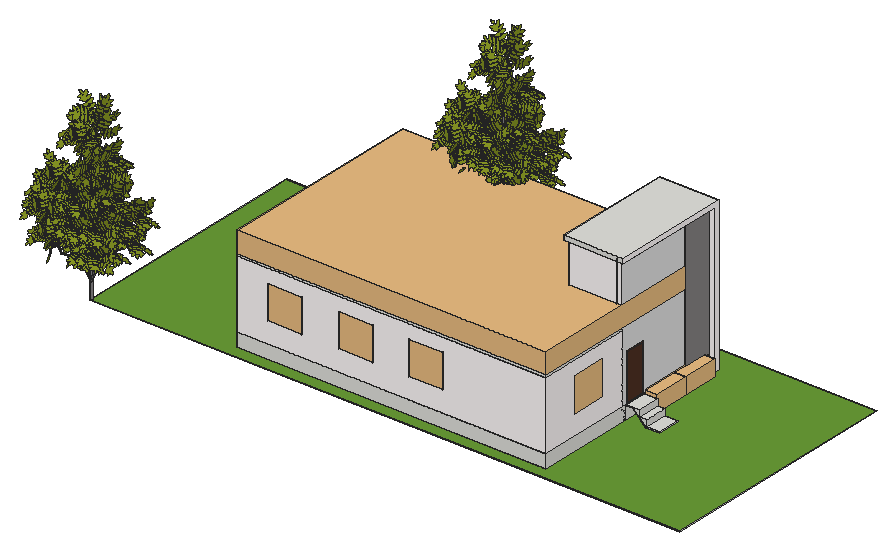
# SketchUp Ruby script. Lengths in inches.
U = 1.inch
M = Sketchup.active_model
def pt(a) = Geom::Point3d.new(a.map { |v| v * U })
def face(e, loops, mat)
  f = e.add_face(loops[0].map { |a| pt(a) })
  loops[1..].each { |l| e.add_face(l.map { |a| pt(a) }).erase! }
  f.material = f.back_material = mat if mat
  f
end
# faces: each face lists its corners as indices into pts; further lists are holes
def faces(e, pts, list, mat = nil) = list.each { |f| face(e, (f[0].is_a?(Array) ? f : [f]).map { |l| l.map { |i| pts[i] } }, mat) }
# xy, xz, yz: faces in a plane at the given z, y or x. An outline is a flat list of corners, or four numbers for a rectangle; further outlines are holes
def ring(l) = l.size == 4 ? [[l[0], l[1]], [l[2], l[1]], [l[2], l[3]], [l[0], l[3]]] : l.each_slice(2).to_a
def flat(e, list, mat, &to3) = list.each { |f| face(e, (f[0].is_a?(Array) ? f : [f]).map { |l| ring(l).map { |u, v| to3.(u, v) } }, mat) }
def xy(e, z, list, mat = nil) = flat(e, list, mat) { |x, y| [x, y, z] }
def xz(e, y, list, mat = nil) = flat(e, list, mat) { |x, z| [x, y, z] }
def yz(e, x, list, mat = nil) = flat(e, list, mat) { |y, z| [x, y, z] }
def lines(e, pts, list) = list.each { |a, b| e.add_line(pt(pts[a]), pt(pts[b])) }
# prism: a flat outline (further loops are holes) pulled along v
def prism(e, loops, v, mat = nil)
  f = face(e, loops, mat); d = Geom::Vector3d.new(v.map { |x| x * U })
  f.pushpull(f.normal.samedirection?(d) ? d.length : -d.length)
end
def box(e, o, s, mat = nil) = prism(e, [[o, [o[0] + s[0], o[1], o[2]], [o[0] + s[0], o[1] + s[1], o[2]], [o[0], o[1] + s[1], o[2]]]], [0, 0, s[2]], mat)
def at(x, y, z, deg = 0) = Geom::Transformation.translation(pt([x, y, z])) * Geom::Transformation.rotation(ORIGIN, Z_AXIS, deg.degrees)
def axes(o, x, y, z) = Geom::Transformation.new([*x, 0, *y, 0, *z, 0, *pt(o).to_a, 1])
def part(name) = M.definitions.add(name)
# library, detail: a bought-in or finely detailed component or shape, given as its bounding box
def library(name, o, s) = part(name).tap { |d| box(d.entities, o, s) }
def detail(e, o, s) = box(e.add_group.entities, o, s)
def put(e, d, t, mat = nil) = e.add_instance(d, t).tap { |i| i.material = mat if mat }
def group(e, t, mat = nil) = e.add_group.tap { |g| g.transformation = t; g.material = mat if mat }.entities
root = M.entities
M.materials.add("3D66_SU_1574822641685_001").color = [135, 150, 36]
M.materials.add("3D66_SU_1574822641883_002").color = [178, 165, 164]
M.materials.add("3D66_SU_1574822642012_003").color = [128, 125, 127]
M.materials.add("Polis06_194").color = [79, 50, 36]
M.materials.add("[0010_Snow]").color = [255, 250, 250]
M.materials.add("[Brick Tumbled]").color = [135, 132, 132]
M.materials.add("[Color M01]").color = [226, 226, 226]
M.materials.add("[Grass Dark Green]").color = [106, 157, 55]
c1 = part("Group7\#1")
p = [[645.1,1113.3,118],[645.1,1115.23,118],[645.1,1197.92,159.125],[645.1,1235.36,159.125],[723.92,1235.36,159.125],[723.92,1197.92,159.125],
  [723.92,1103.42,206.125],[723.92,1091.61,206.125],[680.6,1113.3,118],[680.6,1115.23,118],[680.6,1197.92,159.125],[680.6,1199.86,159.125],
  [688.42,1199.86,159.125],[688.42,1197.92,159.125],[688.42,1103.42,206.125],[688.42,1091.61,206.125]]
lines(c1.entities,p,[[0,1],[1,2],[2,3],[3,4],[4,5],[5,6],[6,7],[8,9],[9,10],[10,11],[11,12],[12,13],
  [13,14],[14,15]])
c2 = part("Group6\#1")
xy(c2.entities,114.0625,[[643.17,1127.05,682.54,1127.97]])
xy(c2.entities,118,[[643.17,1115.23,682.54,1127.05]])
xy(c2.entities,123.875,[[643.17,1127.05,682.54,1138.86]])
xy(c2.entities,129.75,[[643.17,1138.86,682.54,1150.67]])
xy(c2.entities,135.625,[[643.17,1150.67,682.54,1162.48]])
xy(c2.entities,141.5,[[643.17,1162.48,682.54,1174.3]])
xy(c2.entities,147.375,[[643.17,1174.3,682.54,1186.11]])
xy(c2.entities,153.25,[[643.17,1186.11,682.54,1197.92]])
xy(c2.entities,155.1875,[[686.48,1185.18,686.48,1197.92,682.54,1197.92,682.54,1210.66,643.17,1210.66,643.17,1237.3,725.85,1237.3,725.85,1185.18]])
xy(c2.entities,159.125,[[686.48,1186.11,725.85,1186.11,725.85,1237.3,643.17,1237.3,643.17,1197.92,686.48,1197.92]])
xy(c2.entities,165,[[686.48,1174.3,725.85,1186.11]])
xy(c2.entities,170.875,[[686.48,1162.48,725.85,1174.3]])
xy(c2.entities,176.75,[[686.48,1150.67,725.85,1162.48]])
xy(c2.entities,182.625,[[686.48,1138.86,725.85,1150.67]])
xy(c2.entities,188.5,[[686.48,1127.05,725.85,1138.86]])
xy(c2.entities,194.375,[[686.48,1115.23,725.85,1127.05]])
xy(c2.entities,200.25,[[686.48,1103.42,725.85,1115.23]])
xy(c2.entities,206.125,[[686.48,1091.61,725.85,1103.42]])
xz(c2.entities,1103.42,[[686.48,200.25,725.85,206.125]])
xz(c2.entities,1115.23,[[686.48,194.375,725.85,200.25]])
xz(c2.entities,1127.05,[[643.17,118,682.54,123.875],[686.48,188.5,725.85,194.375]])
xz(c2.entities,1138.86,[[643.17,123.875,682.54,129.75],[686.48,182.625,725.85,188.5]])
xz(c2.entities,1150.67,[[643.17,129.75,682.54,135.625],[686.48,176.75,725.85,182.625]])
xz(c2.entities,1162.48,[[643.17,135.625,682.54,141.5],[686.48,170.875,725.85,176.75]])
xz(c2.entities,1174.3,[[643.17,141.5,682.54,147.375],[686.48,165,725.85,170.875]])
xz(c2.entities,1186.11,[[643.17,147.375,682.54,153.25],[686.48,159.125,725.85,165]])
xz(c2.entities,1197.92,[[643.17,153.25,682.54,159.125],[682.54,155.1875,686.48,159.125]])
xz(c2.entities,1237.3,[[643.17,155.1875,725.85,159.125]])
yz(c2.entities,643.17,[[1127.05,114.0625,1127.05,123.875,1138.86,123.875,1138.86,129.75,1150.67,129.75,1150.67,135.625,1162.48,135.625,1162.48,141.5,1174.3,141.5,1174.3,147.375,1186.11,147.375,1186.11,153.25,1197.92,153.25,1197.92,159.125,1237.3,159.125,1237.3,155.1875,1210.66,155.1875,1127.97,114.0625]])
yz(c2.entities,682.54,[[1127.05,114.0625,1127.97,114.0625,1210.66,155.1875,1197.92,155.1875,1197.92,153.25,1186.11,153.25,1186.11,147.375,1174.3,147.375,1174.3,141.5,1162.48,141.5,1162.48,135.625,1150.67,135.625,1150.67,129.75,1138.86,129.75,1138.86,123.875,1127.05,123.875]])
yz(c2.entities,686.48,[[1185.18,155.1875,1090.68,202.1875,1091.61,202.1875,1091.61,206.125,1103.42,206.125,1103.42,200.25,1115.23,200.25,1115.23,194.375,1127.05,194.375,1127.05,188.5,1138.86,188.5,1138.86,182.625,1150.67,182.625,1150.67,176.75,1162.48,176.75,1162.48,170.875,1174.3,170.875,1174.3,165,1186.11,165,1186.11,159.125,1197.92,159.125,1197.92,155.1875]])
yz(c2.entities,725.85,[[1185.18,155.1875,1237.3,155.1875,1237.3,159.125,1186.11,159.125,1186.11,165,1174.3,165,1174.3,170.875,1162.48,170.875,1162.48,176.75,1150.67,176.75,1150.67,182.625,1138.86,182.625,1138.86,188.5,1127.05,188.5,1127.05,194.375,1115.23,194.375,1115.23,200.25,1103.42,200.25,1103.42,206.125,1091.61,206.125,1091.61,202.1875,1090.68,202.1875]])
p = [[643.17,1127.97,114.0625],[643.17,1210.66,155.1875],[682.54,1210.66,155.1875],[682.54,1127.97,114.0625],[725.85,1185.18,155.1875],[725.85,1090.68,202.1875],
  [686.48,1090.68,202.1875],[686.48,1185.18,155.1875]]
faces(c2.entities,p,[[0,1,2,3],[4,5,6,7]])
put(c2.entities,c1,at(0,0,39.375))
c3 = part("Group16\#1")
prism(c3.entities,[[[640.68,60.08,-12.85],[640.68,60.08,-11.85],[640.68,36.46,-11.85],[640.68,36.46,-17.72],[640.68,24.64,-17.72],[640.68,24.64,-23.6],[640.68,1.02,-23.6],[640.68,1.02,-24.6],[640.68,24.88,-24.6],[640.68,48.5,-12.85]]],[-39.375,0,0])
c4 = part("Group\#3")
xy(c4.entities,0,[[0,0,4.72,1.18],[0,34.25,4.72,35.43]],"Polis06_194")
xy(c4.entities,85.26,[[0,1.18,4.72,34.25]],"Polis06_194")
xy(c4.entities,86.61,[[0,0,4.72,35.43]],"Polis06_194")
xz(c4.entities,0,[[0,0,4.72,86.61]],"Polis06_194")
xz(c4.entities,1.18,[[0,0,2.36,85.26],[2.36,0,4.72,85.26]],"Polis06_194")
xz(c4.entities,34.25,[[0,0,4.72,85.26]],"Polis06_194")
xz(c4.entities,35.43,[[0,0,4.72,86.61]],"Polis06_194")
yz(c4.entities,0,[[0,0,1.18,86.61],[34.25,0,35.43,86.61],[1.18,85.26,34.25,86.61]],"Polis06_194")
yz(c4.entities,2.36,[[1.18,0,34.25,0,34.25,85.21,1.18,85.26]],"Polis06_194")
yz(c4.entities,4.72,[[0,0,1.18,86.61],[34.25,0,35.43,86.61],[1.18,85.26,34.25,86.61]],"Polis06_194")
c5 = library("4e1fe49e-2fec-46be-a265-c81cc17eb477",[0,0,0],[35.43,4.93,59.06])
c6 = library("Group\#5",[-532.74,0,0],[536.68,360,36.31])
c7 = library("Group8",[-183.25,9.15,0],[25.91,56.79,43.93])
c8 = part("rama-acacia")
p = [[-13.8,1.01,-1.08],[-13.61,0.91,-1.04],[-13.61,0.85,-1.06],[-14.07,0.85,-1.21],[-15.17,0.86,-1.58],[-15.95,0.92,-1.83],
  [-16.01,1,-1.83],[-16.01,1.17,-1.78],[-16.07,1.93,-1.6],[-16.4,2.73,-1.5],[-16.65,3.06,-1.5],[-17.13,4.01,-1.41],
  [-17.78,4.7,-1.44],[-18.28,5.07,-1.51],[-18.57,5.18,-1.58],[-18.91,5.47,-1.62],[-19.07,5.48,-1.67],[-19.35,5.61,-1.73],
  [-19.51,5.64,-1.78],[-19.38,5.57,-1.75],[-19.33,5.5,-1.75],[-19.31,5.23,-1.82],[-19.38,5.08,-1.89],[-19.41,4.84,-1.96],
  [-19.36,4.59,-2.01],[-19.43,4.55,-2.04],[-19.36,4.15,-2.125],[-19.21,3.7,-2.19],[-18.875,3.1,-2.24],[-18.61,2.78,-2.24],
  [-17.83,2.19,-2.13],[-17.4375,1.85,-2.09],[-17.04,1.49,-2.05],[-16.61,1.24,-1.97],[-16.17,1.0625,-1.87],[-16.06,0.95,-1.86],
  [-16.06,0.91,-1.87],[-16.32,0.9,-1.96],[-16.7,0.88,-2.1],[-17.05,0.91,-2.21],[-17.61,1.15,-2.33],[-18.06,1.29,-2.45],
  [-18.88,1.53,-2.67],[-20.25,1.46,-3.15],[-20.59,1.49,-3.26],[-20.79,1.37,-3.36],[-21.08,1.2,-3.5],[-21.28,1.22,-3.5625],
  [-21.48,0.94,-3.71],[-21.79,0.5,-3.93],[-22.02,0.17,-4.1],[-22.11,0.05,-4.16],[-22.21,-0.02,-4.21],[-22.375,-0.05,-4.28],
  [-22.375,-0.07,-4.28],[-22.18,-0.09,-4.22],[-22.11,-0.07,-4.19],[-21.78,-0.1,-4.09],[-21.6,-0.18,-4.05],[-21.52,-0.27,-4.04],
  [-21.33,-0.33,-4],[-20.94,-0.54,-3.92],[-20.6875,-0.63,-3.86],[-20.54,-0.68,-3.82],[-20.42,-0.67,-3.78],[-20.09,-0.46,-3.61],
  [-19.8,-0.24,-3.45],[-19.21,-0.02,-3.19],[-18.48,0.08,-2.92],[-17.72,0.38,-2.58],[-17.4,0.5,-2.4375],[-16.93,0.75,-2.21],
  [-16.78,0.8,-2.15],[-16.1,0.83,-1.91],[-16.0625,0.81,-1.9],[-16.08,0.77,-1.91],[-16.27,0.72,-1.99],[-16.88,0.39,-2.29],
  [-17.1875,0.15,-2.46],[-17.27,0.02,-2.52],[-17.94,-0.52,-2.89],[-17.94,-0.59,-2.91],[-18.08,-0.68,-2.99],[-18.13,-0.86,-3.05],
  [-18.56,-1.55,-3.38],[-18.71,-2.11,-3.58],[-18.79,-2.61,-3.74],[-18.86,-2.84,-3.83],[-18.87,-3.07,-3.89],[-18.84,-3.22,-3.92],
  [-18.8,-3.26,-3.92],[-18.76,-3.47,-3.96],[-18.76,-3.6,-4],[-18.67,-3.8,-4.02],[-18.61,-3.92,-4.04],[-18.58,-4.11,-4.07],
  [-18.53,-4.18,-4.08],[-18.58,-4.35,-4.14],[-18.65,-4.43,-4.18],[-18.72,-4.51,-4.23],[-18.8125,-4.51,-4.26],[-18.8125,-4.53,-4.26],
  [-18.72,-4.54,-4.24],[-18.66,-4.49,-4.21],[-18.58,-4.43,-4.16],[-18.35,-4.23,-4.03],[-18.32,-4.17,-4],[-18.22,-4.125,-3.95],
  [-18.1,-4,-3.88],[-17.79,-3.72,-3.7],[-17.68,-3.51,-3.61],[-17.32,-3.13,-3.38],[-17.24,-2.94,-3.31],[-16.78,-2.12,-2.93],
  [-16.48,-1.78,-2.73],[-16.3,-1.28,-2.54],[-16.05,-0.75,-2.3125],[-15.89,-0.2,-2.11],[-15.89,0.39,-1.95],[-15.96,0.79,-1.87],
  [-15.91,0.82,-1.84],[-15.27,0.8,-1.63],[-14.18,0.76,-1.27],[-13.78,0.73,-1.15],[-13.78,0.67,-1.16],[-14.23,0.54,-1.35],
  [-14.65,0.33,-1.55],[-14.97,0.02,-1.74],[-15.25,-0.36,-1.9375],[-15.57,-0.72,-2.14],[-15.96,-1.64,-2.52],[-16.2,-2.51,-2.84],
  [-16.2,-3.12,-3],[-16.14,-3.41,-3.06],[-16.1,-3.75,-3.14],[-16.1,-4.09,-3.23],[-16.2,-4.25,-3.3],[-16.2,-4.28,-3.3125],
  [-16.08,-4.19,-3.24],[-15.98,-4.08,-3.18],[-15.96,-3.94,-3.14],[-15.96,-3.8125,-3.1],[-15.9,-3.72,-3.06],[-15.68,-3.55,-2.9375],
  [-15.51,-3.49,-2.86],[-15.3,-3.33,-2.75],[-15.23,-3.17,-2.68],[-15.01,-3.03,-2.57],[-14.875,-2.83,-2.47],[-14.6,-2.59,-2.3125],
  [-14.4,-2.27,-2.16],[-14.12,-1.6,-1.89],[-13.91,-1.1,-1.68],[-13.67,-0.83,-1.53],[-13.53,-0.45,-1.38],[-13.53,0.67,-1.08],
  [-13.53,0.69,-1.07],[-13.38,0.86,-0.98],[-13.38,0.92,-0.96],[-13.32,1.03,-0.91],[-13.32,1.35,-0.82],[-13.28,1.49,-0.77],
  [-13.28,1.99,-0.64],[-13.44,2.67,-0.51],[-13.72,3.31,-0.43],[-13.93,3.71,-0.4],[-14.1,4.39,-0.27],[-14.5625,5.06,-0.25],
  [-14.89,5.62,-0.21],[-15.33,6.1,-0.23],[-15.65,6.8,-0.15],[-15.79,6.89,-0.18],[-15.61,6.52,-0.22],[-15.51,6.32,-0.24],
  [-15.45,6.28,-0.23],[-15.52,6,-0.32],[-15.63,5.6875,-0.45],[-15.77,4.97,-0.68],[-15.7,4.25,-0.85],[-15.46,3,-1.11],
  [-15,2.03,-1.21],[-14.3,1.29,-1.17],[-12.41,6.01,0.65],[-12.44,6.14,0.68],[-12.41,6.29,0.73],[-12.43,6.29,0.73],
  [-12.44,6.26,0.72],[-12.47,6.15,0.68],[-12.49,6.07,0.66],[-12.57,5.75,0.55],[-12.67,5.36,0.43],[-12.79,4.875,0.28],
  [-12.83,4.52,0.18],[-12.83,3.99,0.04],[-12.73,3.11,-0.18],[-12.58,2.52,-0.3125],[-12.3,1.97,-0.41],[-11.88,1.51,-0.46],
  [-11.37,1.0625,-0.48],[-10.75,0.75,-0.45],[-10.75,0.68,-0.47],[-12.55,0.7,-0.79],[-13.21,0.79,-0.89],[-13.2,0.67,-0.92],
  [-12.56,0.62,-0.82],[-11.15,0.56,-0.58],[-10.79,0.54,-0.52],[-10.72,0.52,-0.51],[-10.72,0.5,-0.52],[-10.87,0.47,-0.55],
  [-11.14,0.41,-0.62],[-11.39,0.27,-0.7],[-11.625,-0.01,-0.82],[-11.8,-0.43,-0.96],[-11.83,-0.57,-1],[-12.02,-1.08,-1.17],
  [-12.1,-1.39,-1.27],[-12.17,-1.95,-1.4375],[-12.17,-2.77,-1.65],[-12.09,-3.59,-1.86],[-11.86,-4.26,-2],[-11.8125,-4.4,-2.03],
  [-11.84,-4.49,-2.05],[-11.91,-4.6,-2.1],[-11.97,-4.65,-2.12],[-11.98,-4.67,-2.13],[-11.92,-4.65,-2.11],[-11.84,-4.59,-2.08],
  [-11.77,-4.52,-2.05],[-11.74,-4.47,-2.03],[-11.37,-4.3125,-1.92],[-10.95,-4.0625,-1.78],[-10.82,-3.89,-1.71],[-10.64,-3.57,-1.59],
  [-10.41,-3.05,-1.41],[-10.27,-2.73,-1.3],[-10.07,-1.88,-1.03],[-10.15,-0.71,-0.73],[-10.31,-0.1,-0.6],[-10.5,0.4,-0.5],
  [-10.5,0.48,-0.48],[-10.44,0.53,-0.45],[-10.39,0.64,-0.42],[-10.52,0.73,-0.42],[-10.44,0.93,-0.35],[-10.44,1.2,-0.28],
  [-10.32,1.47,-0.18],[-10.48,2.6875,0.12],[-10.43,2.96,0.2],[-10.75,3.87,0.38],[-11.26,4.93,0.57],[-11.8,5.54,0.64],
  [-12.37,5.93,0.64],[-7.78,0.19,-0.06],[-7.78,0.25,-0.04],[-7.75,0.39,0],[-7.89,0.4,-0.02],[-7.96,0.46,-0.02],
  [-7.96,0.49,-0.01],[-7.76,0.62,0.06],[-7.53,0.99,0.2],[-7.31,1.78,0.45],[-7.31,2.74,0.71],[-7.63,3.6875,0.9],
  [-8.02,4.57,1.07],[-8.66,5.23,1.13],[-8.83,5.4,1.14],[-8.92,5.54,1.16],[-9.1,5.64,1.16],[-9.08,5.6,1.15],
  [-9.02,5.56,1.15],[-8.94,5.46,1.14],[-8.9,5.37,1.12],[-8.9375,5.25,1.08],[-9.14,4.92,0.96],[-9.31,4.5625,0.83],
  [-9.39,3.73,0.6],[-9.44,2.76,0.32],[-9.23,1.59,0.05],[-8.82,0.9,-0.06],[-8.36,0.59,-0.0625],[-8.14,0.51,-0.04],
  [-8.05,0.48,-0.03],[-8.05,0.46,-0.04],[-8.12,0.43,-0.06],[-10.1,0.49,-0.4],[-8.22,0.3125,-0.11],[-8.22,0.25,-0.125],
  [-8.53,0.13,-0.21],[-8.8,-0.16,-0.34],[-8.96,-0.61,-0.49],[-8.96,-0.87,-0.56],[-9.16,-1.42,-0.74],[-9.13,-1.77,-0.83],
  [-9.09,-1.83,-0.84],[-9.125,-1.92,-0.87],[-9.125,-2.13,-0.93],[-9.08,-2.23,-0.95],[-9.15,-2.39,-1],[-9.11,-2.67,-1.07],
  [-9.03,-2.86,-1.11],[-9.07,-3.03,-1.16],[-8.97,-3.23,-1.19],[-8.93,-3.44,-1.24],[-8.93,-3.71,-1.32],[-8.79,-4.05,-1.38],
  [-8.7,-4.25,-1.42],[-8.7,-4.39,-1.46],[-8.76,-4.53,-1.5],[-8.77,-4.65,-1.54],[-8.64,-4.55,-1.49],[-8.27,-4.22,-1.33],
  [-8.1875,-4.06,-1.27],[-8.07,-3.98,-1.23],[-7.98,-3.79,-1.17],[-7.79,-3.59,-1.08],[-7.64,-3.3,-0.97],[-7.64,-3.25,-0.96],
  [-7.59,-3.21,-0.9375],[-7.52,-2.93,-0.85],[-7.52,-2.85,-0.83],[-7.47,-2.81,-0.81],[-7.3,-2.09,-0.59],[-7.32,-2.01,-0.57],
  [-7.27,-1.95,-0.54],[-7.1875,-1.57,-0.42],[-7.17,-1.46,-0.39],[-7.17,-1.16,-0.3125],[-7.23,-0.61,-0.17],[-7.49,-0.15,-0.1],
  [-13.39,-0.07,-1.23],[-13.39,0.25,-1.14],[-13.49,0.5625,-1.09],[-4.5625,0.33,0.09],[-4.22,0.49,0.13],[-4,0.7,0.1875],
  [-3.86,0.99,0.26],[-3.77,1.41,0.38],[-3.7,1.73,0.46],[-3.77,1.99,0.53],[-3.85,2.17,0.58],[-3.88,2.57,0.6875],
  [-3.98,2.9,0.78],[-4.0625,2.97,0.8],[-4.1,3.14,0.84],[-4.1875,3.25,0.87],[-4.27,3.55,0.95],[-4.31,3.71,0.99],
  [-4.42,3.9,1.04],[-4.625,4.2,1.125],[-4.72,4.39,1.18],[-4.89,4.57,1.23],[-4.98,4.73,1.27],[-5,4.72,1.26],
  [-5.01,4.51,1.21],[-4.96,4.32,1.16],[-4.97,4.27,1.14],[-5.14,3.78,1.01],[-5.3,3.39,0.91],[-5.44,2.76,0.74],
  [-5.5,2.09,0.56],[-5.57,1.78,0.48],[-5.57,1.42,0.38],[-5.57,1.09,0.29],[-5.47,0.72,0.19],[-5.22,0.44,0.12],
  [-4.93,0.27,0.07],[-4.76,0.22,0.06],[-4.76,0.18,0.05],[-4.83,0.16,0.04],[-5.26,0,0],[-5.34,-0.04,-0.01],
  [-5.47,-0.22,-0.06],[-5.51,-0.6,-0.16],[-5.42,-1.09,-0.29],[-5.28,-1.49,-0.4],[-5.21,-1.87,-0.5],[-5.11,-2.15,-0.57],
  [-5.08,-2.34,-0.63],[-5.01,-2.47,-0.66],[-4.96,-2.69,-0.72],[-4.86,-2.9375,-0.79],[-4.84,-3.07,-0.82],[-4.77,-3.18,-0.85],
  [-4.74,-3.43,-0.92],[-4.7,-3.71,-0.99],[-4.62,-3.89,-1.04],[-4.58,-3.98,-1.07],[-4.58,-3.83,-1.03],[-4.51,-3.67,-0.98],
  [-4.3,-3.32,-0.89],[-4.16,-3.09,-0.83],[-4.16,-2.98,-0.8],[-4.11,-2.92,-0.78],[-4.02,-2.8,-0.75],[-3.95,-2.59,-0.69],
  [-3.95,-2.33,-0.625],[-3.86,-2.26,-0.6],[-3.86,-2.02,-0.54],[-3.86,-1.44,-0.39],[-3.94,-1.22,-0.33],[-3.94,-1.08,-0.29],
  [-4,-0.96,-0.26],[-4,-0.87,-0.23],[-4.0625,-0.8125,-0.22],[-4.16,-0.54,-0.14],[-4.39,-0.24,-0.06],[-4.61,-0.08,-0.02],
  [-4.77,-0.03,-0.01],[-4.77,-0.01,0],[-4.65,-0.01,0],[-4.61,0.19,0.05],[-4.66,0.23,0.0625],[-4.63,0.29,0.08],
  [-4.07,0.17,0.04],[0,-0.24,-0.06],[0,0,0],[-0.5,0.04,0.01],[-1.58,0.08,0.02]]
faces(c8.entities,p,[[0,1,2,3,4,5,6,7,8,9,10,11,12,13,14,15,16,17,18,19,20,21,22,23,24,25,26,27,28,29,30,31,32,33,34,35,36,37,38,39,40,41,42,43,44,45,46,47,48,49,50,51,52,53,54,55,56,57,58,59,60,61,62,63,64,65,66,67,68,69,70,71,72,73,74,75,76,77,78,79,80,81,82,83,84,85,86,87,88,89,90,91,92,93,94,95,96,97,98,99,100,101,102,103,104,105,106,107,108,109,110,111,112,113,114,115,116,117,118,119,120,121,122,123,124,125,126,127,128,129,130,131,132,133,134,135,136,137,138,139,140,141,142,143,144,145,146,147,148,149,150,151,152,153,154,155,156,157,158,159,160,161,162,163,164,165,166,167,168,169,170,171,172,173,174,175,176,177,178,179,180,181],[182,183,184,185,186,187,188,189,190,191,192,193,194,195,196,197,198,199,200,201,202,203,204,205,206,207,208,209,210,211,212,213,214,215,216,217,218,219,220,221,222,223,224,225,226,227,228,229,230,231,232,233,234,235,236,237,238,239,240,241,242,243,244,245,246,247,248,249,250,251,252],[253,254,255,256,257,258,259,260,261,262,263,264,265,266,267,268,269,270,271,272,273,274,275,276,277,278,279,280,281,282,283,284,242,241,285,286,287,288,289,290,291,292,293,294,295,296,297,298,299,300,301,302,303,304,305,306,307,308,309,310,311,312,313,314,315,316,317,318,319,320,321,322,323,324,325,326,327,328,329],[154,330,331,332,155],[333,334,335,336,337,338,339,340,341,342,343,344,345,346,347,348,349,350,351,352,353,354,355,356,357,358,359,360,361,362,363,364,365,366,367,368,369,370,371,372,373,374,375,376,377,378,379,380,381,382,383,384,385,386,387,388,389,390,391,392,393,394,395,396,397,398,399,400,401,402,403,404,405,406,407,408,409,410,411,412,413],[156,203,157],[202,157,203],[414,411,410,415,416,417,418],
  [254,370,255],[369,255,370]],"3D66_SU_1574822641685_001")
c9 = part("ramas")
put(c9.entities,c8,axes([0.11,0.06,-0.22],[-0.42655,-0.79206,-0.43668],[0.22445,0.37501,-0.89944],[0.87617,-0.48167,0.01782]))
put(c9.entities,c8,axes([0.14,0.21,0.02],[0.24321,-0.08852,-0.96593],[0.34202,0.93969,0],[0.90767,-0.33037,0.25882]))
put(c9.entities,c8,at(0,0.24,0.06))
put(c9.entities,c8,axes([0.11,0.45,0.57],[-0.42655,0.68302,0.5929],[0.22445,-0.55509,0.80093],[0.87617,0.47472,0.08347]))
put(c9.entities,c8,axes([0.11,0.73,0.01],[-0.42655,0.88928,-0.16503],[0.22445,0.28083,0.93314],[0.87617,0.36099,-0.31939]))
c10 = part("rama principal")
put(c10.entities,c8,axes([-20.25,-0.15,12.84],[0.38818,-0.89018,-0.23852],[0.89018,0.42916,-0.15296],[0.23852,-0.15296,0.95902]))
put(c10.entities,c8,at(-20.48,0,12.88))
put(c10.entities,c8,axes([-20.6875,-0.1,12.85],[0.57358,0.79124,0.21201],[-0.79124,0.60214,-0.10661],[-0.21201,-0.10661,0.97144]))
put(c10.entities,c8,axes([-20.375,-0.01,13.02],[-0.37792,0.77975,-0.49916],[-0.65887,0.15226,0.73669],[0.65043,0.60729,0.45621]))
put(c10.entities,c8,axes([-20.34,-0.04,12.83],[0.24321,-0.08852,-0.96593],[0.34202,0.93969,0],[0.90767,-0.33037,0.25882]))
put(c10.entities,c8,axes([-20.375,-0.18,12.6],[-0.42655,-0.79206,-0.43668],[0.22445,0.37501,-0.89944],[0.87617,-0.48167,0.01782]))
put(c10.entities,c9,at(-11.43,0,7.77))
g1 = group(c10.entities,at(0,0.2,0),"3D66_SU_1574822641883_002")
xz(g1,0.1,[[-0.15,-0.08,-3.26,5.59,-11.5,7.61,-18.23,12.71,-20.48,12.71,-20.48,13.05,-18.11,13.05,-11.35,7.92,-3.03,5.89,0.15,0.08]])
yz(g1,-20.48,[[0.1,12.71,-0.2,12.88,0.1,13.05]])
p = [[-0.15,0.1,-0.08],[0,-0.2,0],[-3.15,-0.2,5.74],[-3.26,0.1,5.59],[0.15,0.1,0.08],[-3.03,0.1,5.89],
  [-11.43,-0.2,7.77],[-11.5,0.1,7.61],[-11.35,0.1,7.92],[-18.17,-0.2,12.88],[-18.23,0.1,12.71],[-18.11,0.1,13.05],
  [-20.48,-0.2,12.88],[-20.48,0.1,12.71],[-20.48,0.1,13.05]]
faces(g1,p,[[0,1,2,3],[0,4,1],[1,4,5,2],[3,2,6,7],[2,5,8,6],[7,6,9,10],[6,8,11,9],[10,9,12,13],
  [9,11,14,12]])
c11 = part("Component\#1")
p = [[44.23,0.79,16.51],[35.57,0.79,41.625],[19.17,0.79,51.61],[7.37,0.79,32.7],[0.16,0.79,57.85],[31.31,0.79,23.98]]
lines(c11.entities,p,[[0,1],[1,2],[3,4],[5,3]])
g2 = group(c11.entities,at(44.23,0.79,-28.39))
xz(g2,0.2,[[-0.32,44.79,-8.95,69.78,-25.24,79.7,-24.89,80.28,-8.38,70.24,0.32,45.01]],"3D66_SU_1574822642012_003")
p = [[-0.32,0.2,44.79],[0,-0.39,44.9],[-8.67,-0.39,70.01],[-8.95,0.2,69.78],[0.32,0.2,45.01],[-8.38,0.2,70.24],
  [-25.06,-0.39,79.99],[-25.24,0.2,79.7],[-24.89,0.2,80.28]]
faces(g2,p,[[0,1,2,3],[0,4,1],[1,4,5,2],[3,2,6,7],[2,5,8,6],[8,7,6]],"3D66_SU_1574822642012_003")
g3 = group(c11.entities,at(44.23,0.79,-28.39),"3D66_SU_1574822642012_003")
p = [[-0.6,0.39,28.39],[0,-0.79,28.71],[-12.89,-0.52,52.37],[-13.25,0.19,52.17],[0.6,0.39,29.04],[-12.53,0.19,52.57]]
faces(g3,p,[[0,1,2,3],[4,0,3,5],[1,4,5,2]],"3D66_SU_1574822642012_003")
faces(g3,p,[[0,4,1],[5,3,2]])
g4 = group(c11.entities,at(44.23,0.79,-28.39))
prism(g4,[[[-37.03,0.1,61.04],[-36.7,0.1,61.13],[-36.86,-0.2,61.08]]],[-7.21,0,25.15],"3D66_SU_1574822642012_003")
g5 = group(c11.entities,at(44.23,0.79,-28.39))
prism(g5,[[[-13.04,0.2,52.05],[-12.81,0.2,52.69],[-12.92,-0.39,52.37]]],[-23.94,0,8.71],"3D66_SU_1574822642012_003")
c12 = part("Group\#7")
p = [[74.89,60.42,11.53],[61.97,60.42,35.1875]]
lines(c12.entities,p,[[0,1]])
put(c12.entities,c10,at(68.97,49.02,23.76))
put(c12.entities,c10,at(53.09,47.85,77.85))
put(c12.entities,c10,at(71.03,52.76,41.54))
put(c12.entities,c11,at(57.21,20.01,0,65))
put(c12.entities,c11,at(36.98,37.62,26.03,30))
put(c12.entities,c10,at(64.15,37.99,51.46))
put(c12.entities,c10,at(56.21,20.74,57.94))
put(c12.entities,c10,at(58.92,27.24,32.75))
put(c12.entities,c10,at(63.69,53.97,50.16))
put(c12.entities,c10,at(67.38,56.1,67.8))
put(c12.entities,c10,at(42.86,42.51,58.92))
c13 = part("Group\#15")
put(c13.entities,c10,axes([77.34,81.85,135.3],[0.74154,0,-1.06776],[0,1.3,0],[1.06776,0,0.74154]))
put(c13.entities,c10,axes([75.32,76.01,111.65],[-0.93342,-0.35878,0],[0,0,1],[-0.35878,0.93342,0]))
put(c13.entities,c10,at(75.26,75.24,133.54))
put(c13.entities,c10,at(86.81,70.77,127.28,-169.088))
put(c13.entities,c10,axes([74.83,76.55,119.32],[0.01789,-0.99984,0],[0,0,1],[-0.99984,-0.01789,0]))
put(c13.entities,c10,axes([74.58,75.83,133.24],[0.00428,0.99999,0],[0,0,1],[0.99999,-0.00428,0]))
g6 = group(c13.entities,at(74.89,76.17,0))
xy(g6,28.71,[[-0.95,-1.375,-0.95,1.51,1.75,0.07]])
xy(g6,61.08,[[-0.46,-0.98,1.24,0,-0.46,0.98]])
p = [[-0.95,1.51,28.71],[-0.95,-1.375,28.71],[-0.46,0.98,61.08],[1.75,0.07,28.71],[1.57,0,36.81],[-0.79,-1.36,36.81],
  [-0.79,1.36,36.81],[-0.79,1.36,44.9],[1.57,0,44.9],[-0.79,-1.36,44.9],[1.24,0,61.08],[-0.46,-0.98,61.08]]
faces(g6,p,[[0,1,2],[3,4,1],[1,4,5],[1,5,2],[4,3,6],[0,6,3],[2,0,7],[6,7,0],
  [4,8,9,5],[9,2,5],[6,7,8,4],[8,10,11,9],[11,2,9],[7,2,10,8]],"3D66_SU_1574822642012_003")
g7 = group(c13.entities,at(74.89,76.17,0),"3D66_SU_1574822642012_003")
xy(g7,0,[[-0.98,-1.7,-0.98,1.7,1.97,0]])
xy(g7,28.71,[[-0.78,-1.47,1.76,0,-0.78,1.47]])
p = [[1.97,0,0],[1.76,0,28.71],[-0.78,-1.47,28.71],[-0.98,-1.7,0],[-0.78,1.47,28.71],[-0.98,1.7,0]]
faces(g7,p,[[0,1,2,3],[2,4,5,3],[5,4,1,0]])
put(c13.entities,c12,at(23.47,157.51,17.18,-96.594))
put(c13.entities,c12,at(0,15.76,17.18))
put(c13.entities,c12,at(169.96,91.05,17.18,150))
put(c13.entities,c12,at(128.55,-3.7,17.18,85))
g8 = group(c13.entities,at(75.13,76.19,0))
xy(g8,61.08,[[-0.7,-0.96,-0.7,0.96,1,0]],"3D66_SU_1574822642012_003")
xy(g8,133.54,[[-0.3,-0.51,0.6,0,-0.3,0.51]],"3D66_SU_1574822642012_003")
p = [[-0.3,-0.51,133.54],[-0.3,0.51,133.54],[-0.7,0.96,61.08],[-0.7,-0.96,61.08],[1,0,61.08],[0.6,0,133.54]]
faces(g8,p,[[0,1,2,3],[4,5,0,3],[2,1,5,4]],"3D66_SU_1574822642012_003")
xy(root,-24.1,[[96.82,90.85,1120.4,472.81]])
xy(root,-23.6,[[96.82,90.85,1120.4,518.11]],"[Grass Dark Green]")
xy(root,239.94,[[779.5,266.28,882.86,473.59]])
xz(root,90.85,[[96.82,-24.1,1120.4,-23.6]])
xz(root,266.28,[[779.5,231.94,882.8,239.94]])
xz(root,473.59,[[779.5,236,882.86,239.94]])
yz(root,96.82,[[90.85,-24.1,90.85,-23.6,518.11,-23.6,472.81,-24.1]])
yz(root,779.5,[[266.28,231.94,266.28,239.94,473.59,239.94,473.59,236]])
yz(root,871.06,[[286.08,231.94,465.59,236]])
yz(root,1120.4,[[90.85,-24.1,472.81,-24.1,518.11,-23.6,90.85,-23.6]])
# 10 loose lines left out
p = [[96.82,518.11,-23.6],[1120.4,518.11,-23.6],[1120.4,472.81,-24.1],[96.82,472.81,-24.1]]
faces(root,p,[[0,1,2,3]])
g9 = group(root,at(334.375,113.59,0),"[0010_Snow]")
xy(g9,-23.6,[[536.68,352,548.48,360]])
xy(g9,0,[[0,0,0,360,528.14,360,528.14,349.125,450.875,349.125,450.875,208.61,445.13,208.61,445.13,349.125,157.8,349.125,157.8,225.1875,150.33,225.1875,150.33,230.78,152.05,230.78,152.05,349.125,10.58,349.125,10.58,230.78,113.11,230.78,113.11,225.1875,110.03,225.1875,110.03,201.57,104.59,201.57,104.59,225.1875,10.58,225.1875,10.58,170.33,104.59,170.33,104.59,171.88,110.03,171.88,110.03,170.33,113.76,170.33,113.76,164.2,10.58,164.2,10.58,9.4375,152.05,9.4375,152.05,164.2,150.07,164.2,150.07,170.33,203.14,170.33,203.14,164.2,157.72,164.2,157.72,9.4375,256.35,9.4375,256.35,164.49,251.29,164.49,251.29,170.33,354.04,170.33,354.04,164.49,261.37,164.49,261.37,9.4375,392.31,9.4375,392.31,170.33,400.41,170.33,400.41,164.49,397.5,164.49,397.5,9.4375,528.5,9.4375,528.5,164.49,536.68,164.49,536.68,0],[435.46,164.49,528.5,170.33]])
xy(g9,0,[[536.68,301.66,537.68,349.125],[528.14,349.125,536.68,352],[536.68,349.125,537.68,352]],"[Color M01]")
xy(g9,35.43,[[52.96,0,113.1,9.4375],[176.51,0,235.97,9.4375],[298.47,0,358.21,9.4375],[528.5,60.51,536.68,120.22],[54.3,349.125,113.03,360],
  [180.36,349.125,239.71,360],[365.54,349.125,424.86,360],[465.84,349.125,512.28,360]])
xy(g9,70.8,[[0,189.26,10.58,206.83]])
xy(g9,82.6,[[113.76,164.2,150.07,170.33],[354.04,164.49,392.31,170.33],[400.41,164.49,435.46,170.33],[445.13,170.33,450.875,208.61],[104.59,171.88,110.03,201.57],
  [113.11,225.1875,150.33,230.78]])
xy(g9,94.4,[[0,189.26,10.58,206.83]])
xy(g9,94.43,[[52.96,0,113.1,9.4375],[176.51,0,235.97,9.4375],[298.47,0,358.21,9.4375],[528.5,60.51,536.68,120.22],[54.3,349.125,113.03,360],
  [180.36,349.125,239.71,360],[365.54,349.125,424.86,360],[465.84,349.125,512.28,360]])
xy(g9,118,[[[0,0,52.96,0,52.96,9.4375,10.58,9.4375,10.58,164.2,152.05,164.2,152.05,9.4375,113.1,9.4375,113.1,0,176.51,0,176.51,9.4375,157.72,9.4375,157.72,164.2,203.14,164.2,203.14,170.33,110.03,170.33,110.03,225.1875,157.8,225.1875,157.8,349.125,445.13,349.125,445.13,360,0,360],[10.58,230.78,152.05,349.125],[10.58,170.33,104.59,225.1875]],[52.96,0,113.1,9.4375],[[176.51,0,536.68,0,536.68,164.49,528.5,164.49,528.5,9.4375,397.5,9.4375,397.5,164.49,445.13,164.49,445.13,170.33,251.29,170.33,251.29,164.49,256.35,164.49,256.35,9.4375,176.51,9.4375],[261.37,9.4375,392.31,164.49]]])
xy(g9,231.94,[[536.68,152.6875,548.48,172.49],[536.68,172.49,536.68,301.66,537.68,301.66,537.68,352,548.48,352,548.48,172.49]])
xy(g9,236,[[445.13,164.49,528.5,164.49,528.5,170.33,450.875,170.33,450.875,349.125,528.14,349.125,528.5,360,445.13,360]])
xz(g9,0,[[[0,0,536.68,118],[52.96,35.43,113.1,94.43],[298.47,35.43,358.21,94.43],[176.51,35.43,235.97,94.43]]])
xz(g9,9.4375,[[[10.58,0,152.05,118],[52.96,35.43,113.1,94.43]],[[157.72,0,256.35,118],[176.51,35.43,235.97,94.43]],[[261.37,0,392.31,118],[298.47,35.43,358.21,94.43]],[397.5,0,528.5,118]])
xz(g9,60.51,[[528.5,35.43,536.68,94.43]])
xz(g9,120.22,[[528.5,35.43,536.68,94.43]])
xz(g9,164.2,[[10.58,0,113.76,0,113.76,82.6,150.07,82.6,150.07,0,152.05,0,152.05,118,10.58,118],[157.72,0,203.14,118]])
xz(g9,164.49,[[251.29,0,256.35,118],[261.37,0,354.04,0,354.04,82.6,392.31,82.6,392.31,118,261.37,118],[397.5,0,400.41,0,400.41,82.6,435.46,82.6,435.46,0,528.5,0,528.5,236,445.13,236,445.13,118,397.5,118],[528.5,0,536.68,118],[528.5,118,536.68,236]])
xz(g9,170.33,[[10.58,0,104.59,118],[110.03,0,110.03,118,203.14,118,203.14,0,150.07,0,150.07,82.6,113.76,82.6,113.76,0],[251.29,0,251.29,118,445.13,118,445.13,82.6,450.875,82.6,450.875,0,435.46,0,435.46,82.6,400.41,82.6,400.41,0,392.31,0,392.31,82.6,354.04,82.6,354.04,0],[450.875,0,528.5,236]])
xz(g9,171.88,[[104.59,0,110.03,82.6]])
xz(g9,189.26,[[0,70.8,10.58,94.4]])
xz(g9,201.57,[[104.59,0,110.03,82.6]])
xz(g9,206.83,[[0,70.8,10.58,94.4]])
xz(g9,208.61,[[445.13,0,450.875,82.6]])
xz(g9,225.1875,[[10.58,0,104.59,118],[110.03,0,113.11,0,113.11,82.6,150.33,82.6,150.33,0,157.8,0,157.8,118,110.03,118]])
xz(g9,230.78,[[10.58,0,10.58,118,152.05,118,152.05,0,150.33,0,150.33,82.6,113.11,82.6,113.11,0]])
xz(g9,301.66,[[536.68,0,537.68,231.94]],"[Color M01]")
xz(g9,349.125,[[[10.58,0,152.05,118],[54.3,35.43,113.03,94.43]],[[157.8,0,445.13,118],[180.36,35.43,239.71,94.43],[365.54,35.43,424.86,94.43]],[[450.875,0,528.14,236],[465.84,35.43,512.28,94.43]]])
xz(g9,352,[[536.68,-23.6,548.48,-23.6,548.48,231.94,537.68,231.94,537.68,0,536.68,0]])
xz(g9,360,[[536.68,-23.6,536.68,236,548.48,239.94,548.48,-23.6],[528.5,-0.75,528.14,0,528.5,0],[528.5,-0.75,536.68,236],[[0,0,0,118,445.13,118,445.13,236,528.5,236,528.5,0],[180.36,35.43,239.71,94.43],[365.54,35.43,424.86,94.43],[54.3,35.43,113.03,94.43],[465.84,35.43,512.28,94.43]]])
yz(g9,0,[[[0,0,360,118],[189.26,70.8,206.83,94.4]]])
yz(g9,10.58,[[9.4375,0,164.2,118],[[170.33,0,225.1875,118],[189.26,70.8,206.83,94.4]],[230.78,0,349.125,118]])
yz(g9,52.96,[[0,35.43,9.4375,94.43]])
yz(g9,54.3,[[349.125,35.43,360,94.43]])
yz(g9,104.59,[[170.33,0,170.33,118,225.1875,118,225.1875,0,201.57,0,201.57,82.6,171.88,82.6,171.88,0]])
yz(g9,110.03,[[170.33,0,171.88,0,171.88,82.6,201.57,82.6,201.57,0,225.1875,0,225.1875,118,170.33,118]])
yz(g9,113.03,[[349.125,35.43,360,94.43]])
yz(g9,113.1,[[0,35.43,9.4375,94.43]])
yz(g9,113.11,[[225.1875,0,230.78,82.6]])
yz(g9,113.76,[[164.2,0,170.33,82.6]])
yz(g9,150.07,[[164.2,0,170.33,82.6]])
yz(g9,150.33,[[225.1875,0,230.78,82.6]])
yz(g9,152.05,[[9.4375,0,164.2,118],[230.78,0,349.125,118]])
yz(g9,157.72,[[9.4375,0,164.2,118]])
yz(g9,157.8,[[225.1875,0,349.125,118]])
yz(g9,176.51,[[0,35.43,9.4375,94.43]])
yz(g9,180.36,[[349.125,35.43,360,94.43]])
yz(g9,203.14,[[164.2,0,170.33,118]])
yz(g9,235.97,[[0,35.43,9.4375,94.43]])
yz(g9,239.71,[[349.125,35.43,360,94.43]])
yz(g9,251.29,[[164.49,0,170.33,118]])
yz(g9,256.35,[[9.4375,0,164.49,118]])
yz(g9,261.37,[[9.4375,0,164.49,118]])
yz(g9,298.47,[[0,35.43,9.4375,94.43]])
yz(g9,354.04,[[164.49,0,170.33,82.6]])
yz(g9,358.21,[[0,35.43,9.4375,94.43]])
yz(g9,365.54,[[349.125,35.43,360,94.43]])
yz(g9,392.31,[[9.4375,0,9.4375,118,164.49,118,164.49,82.6,170.33,82.6,170.33,0]])
yz(g9,397.5,[[9.4375,0,164.49,118]])
yz(g9,400.41,[[164.49,0,170.33,82.6]])
yz(g9,424.86,[[349.125,35.43,360,94.43]])
yz(g9,435.46,[[164.49,0,170.33,82.6]])
yz(g9,445.13,[[208.61,0,208.61,82.6,170.33,82.6,170.33,236,349.125,236,349.125,0],[164.49,118,170.33,236],[349.125,118,360,236]])
yz(g9,450.875,[[208.61,0,349.125,0,349.125,236,170.33,236,170.33,82.6,208.61,82.6]])
yz(g9,465.84,[[349.125,35.43,360,94.43]])
yz(g9,512.28,[[349.125,35.43,360,94.43]])
yz(g9,528.14,[[349.125,0,360,0,349.125,118]])
yz(g9,528.5,[[[9.4375,0,164.49,118],[60.51,35.43,120.22,94.43]],[164.49,0,170.33,236]])
yz(g9,536.68,[[164.49,-23.6,172.12,0],[172.12,-23.6,172.15,0,172.12,0],[301.66,-23.6,352,0],[352,-23.6,360,0],[[0,0,164.49,118],[60.51,35.43,120.22,94.43]],
  [301.66,0,301.66,231.94,170.33,231.94,170.33,236,360,236,360,0],[172.12,0,172.15,0,172.15,2.67],[152.6875,231.94,164.49,236],[164.49,231.94,170.33,236]])
yz(g9,536.68,[[164.49,0,164.49,231.94,301.66,231.94,301.66,0,212.49,0,212.49,82.6,173.3,82.6,172.15,2.67,172.12,0]],"[Color M01]")
yz(g9,537.68,[[301.66,0,352,231.94]],"[Brick Tumbled]")
yz(g9,548.48,[[352,-23.6,360,-23.6,360,239.94,152.6875,239.94,152.6875,231.94,352,231.94]])
# 4 loose lines left out
p = [[528.5,360,-0.75],[528.14,349.125,118],[528.14,360,0],[528.5,360,0],[528.5,360,236],[528.14,349.125,236]]
faces(g9,p,[[0,1,2],[1,0,3,4,5]])
put(g9,c2,at(-178.6,-899.1875,-114.0625,0.881))
g10 = group(root,at(334.375,113.59,-23.6))
xy(g10,0,[[0,0,536.68,359.22]])
xy(g10,23.6,[[0,0,536.68,359.22]])
xz(g10,0,[[0,0,536.68,23.6]])
xz(g10,359.22,[[0,0,536.68,23.6]])
yz(g10,0,[[0,0,359.22,23.6]])
yz(g10,536.68,[[0,0,172.12,23.6],[172.12,0,212.49,23.6],[212.49,0,359.22,23.6]])
# 2 loose lines left out
put(g10,c3,axes([596.77,-428.2,45.53],[0,1,0],[-1,0,0],[0,0,1.85098]))
put(root,c4,axes([780.52,282.39,0],[1,0,0],[0,1.12351,0],[0,0,0.95365]))
put(root,c4,axes([448.13,283.91,0],[-0.03128,-0.59692,0],[1.02201,-0.05356,0],[0,0,0.95365]))
put(root,c4,axes([688.41,283.91,0],[-0.03015,-0.57528,0],[1.07707,-0.05645,0],[0,0,0.95365]))
put(root,c4,axes([734.79,283.91,0],[-0.03202,-0.61095,0],[0.98632,-0.05169,0],[0,0,0.95365]))
put(root,c4,axes([439.68,285.47,0],[1,0,0],[0,0.83788,0],[0,0,0.95365]))
g11 = group(root,at(334.375,113.59,118))
xy(g11,0,[[0,0,0,360,446.44,360,446.44,163.875,536.68,163.875,536.68,0]])
xy(g11,3.94,[[0,0,536.68,0,536.68,163.875,446.44,163.875,446.44,360,0,360]])
xz(g11,0,[[0,0,536.68,3.94]])
xz(g11,163.875,[[446.44,0,536.68,3.94]])
xz(g11,360,[[0,0,446.44,3.94]])
yz(g11,0,[[0,0,360,3.94]])
yz(g11,446.44,[[163.875,0,168.8125,3.94],[168.8125,0,360,3.94]])
yz(g11,536.68,[[0,0,163.875,3.94]])
# 1 loose lines left out
put(root,c5,axes([632.85,113.59,35.43],[1.68604,0,0],[0,1,0],[0,0,1]))
put(root,c5,axes([510.89,113.59,35.43],[1.68604,0,0],[0,1,0],[0,0,1]))
put(root,c5,axes([387.34,113.59,35.43],[1.68604,0,0],[0,1,0],[0,0,1]))
put(root,c5,axes([867.12,233.8125,35.43],[0,-1.68604,0],[1,0,0],[0,0,1]))
put(root,c6,at(867.12,113.59,121.94))
put(root,c4,axes([866.33,286.26,0],[1,0,0],[0,1.12351,0],[0,0,0.95365]))
put(root,c5,axes([800.21,469.65,35.43],[1.31071,0,0],[0,0.79898,0],[0,0,1]))
put(root,c5,axes([514.73,469.65,35.43],[1.68604,0,0],[0,1,0],[0,0,1]))
put(root,c5,axes([387.73,469.65,35.43],[1.68604,0,0],[0,1,0],[0,0,1]))
put(root,c5,axes([699.88,469.65,35.43],[1.68604,0,0],[0,1,0],[0,0,1]))
put(root,c7,axes([1016.47,400.96,-23.6],[0.79351,0,0],[0,-1.10365,0],[0,0,0.6372]))
put(root,c7,axes([1016.47,464.34,-23.6],[0.79351,0,0],[0,-1.10365,0],[0,0,0.6372]))
put(root,c13,axes([398.27,395.21,50.32],[1.31,0,0],[0,1.22,0],[0,0,1.6799]))
put(root,c13,axes([0,0,-24.1],[1.31,0,0],[0,1.22,0],[0,0,1.6799]))
